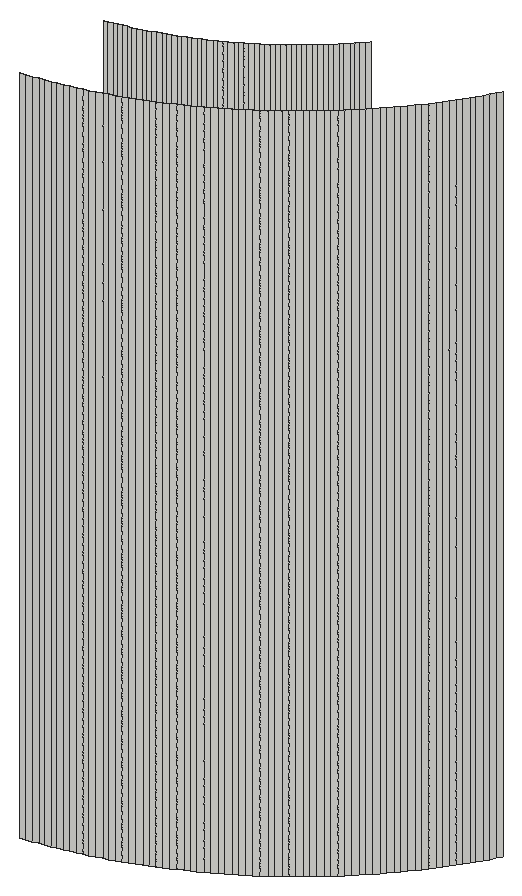
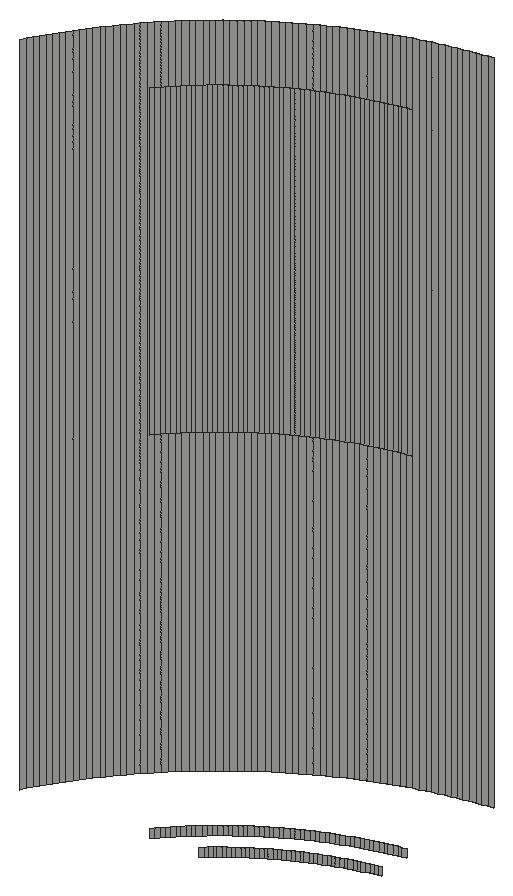
# SketchUp Ruby script. Lengths in inches.
U = 1.inch
M = Sketchup.active_model
def pt(a) = Geom::Point3d.new(a.map { |v| v * U })
def face(e, loops, mat)
  f = e.add_face(loops[0].map { |a| pt(a) })
  loops[1..].each { |l| e.add_face(l.map { |a| pt(a) }).erase! }
  f.material = f.back_material = mat if mat
  f
end
# faces: each face lists its corners as indices into pts; further lists are holes
def faces(e, pts, list, mat = nil) = list.each { |f| face(e, (f[0].is_a?(Array) ? f : [f]).map { |l| l.map { |i| pts[i] } }, mat) }
# xy, xz, yz: faces in a plane at the given z, y or x. An outline is a flat list of corners, or four numbers for a rectangle; further outlines are holes
def ring(l) = l.size == 4 ? [[l[0], l[1]], [l[2], l[1]], [l[2], l[3]], [l[0], l[3]]] : l.each_slice(2).to_a
def flat(e, list, mat, &to3) = list.each { |f| face(e, (f[0].is_a?(Array) ? f : [f]).map { |l| ring(l).map { |u, v| to3.(u, v) } }, mat) }
def xy(e, z, list, mat = nil) = flat(e, list, mat) { |x, y| [x, y, z] }
def xz(e, y, list, mat = nil) = flat(e, list, mat) { |x, z| [x, y, z] }
def yz(e, x, list, mat = nil) = flat(e, list, mat) { |y, z| [x, y, z] }
def lines(e, pts, list) = list.each { |a, b| e.add_line(pt(pts[a]), pt(pts[b])) }
# prism: a flat outline (further loops are holes) pulled along v
def prism(e, loops, v, mat = nil)
  f = face(e, loops, mat); d = Geom::Vector3d.new(v.map { |x| x * U })
  f.pushpull(f.normal.samedirection?(d) ? d.length : -d.length)
end
def box(e, o, s, mat = nil) = prism(e, [[o, [o[0] + s[0], o[1], o[2]], [o[0] + s[0], o[1] + s[1], o[2]], [o[0], o[1] + s[1], o[2]]]], [0, 0, s[2]], mat)
def at(x, y, z, deg = 0) = Geom::Transformation.translation(pt([x, y, z])) * Geom::Transformation.rotation(ORIGIN, Z_AXIS, deg.degrees)
def axes(o, x, y, z) = Geom::Transformation.new([*x, 0, *y, 0, *z, 0, *pt(o).to_a, 1])
def part(name) = M.definitions.add(name)
# library, detail: a bought-in or finely detailed component or shape, given as its bounding box
def library(name, o, s) = part(name).tap { |d| box(d.entities, o, s) }
def detail(e, o, s) = box(e.add_group.entities, o, s)
def put(e, d, t, mat = nil) = e.add_instance(d, t).tap { |i| i.material = mat if mat }
def group(e, t, mat = nil) = e.add_group.tap { |g| g.transformation = t; g.material = mat if mat }.entities
root = M.entities
p = [[327.44,164.25,231],[327.44,164.25,270],[327.13,164.21,270],[327.13,164.21,231],[327.75,164.3,231],[327.75,164.3,270],
  [328.0625,164.35,231],[328.0625,164.35,270],[328.375,164.4,231],[328.375,164.4,270],[328.68,164.46,231],[328.68,164.46,270],
  [328.99,164.52,231],[328.99,164.52,270],[329.3,164.59,231],[329.3,164.59,270],[329.6,164.66,231],[329.6,164.66,270],
  [329.91,164.74,231],[329.91,164.74,270],[330.21,164.82,231],[330.21,164.82,270],[330.51,164.9,231],[330.51,164.9,270],
  [330.82,164.99,231],[330.82,164.99,270],[331.12,165.08,231],[331.12,165.08,270],[331.42,165.17,231],[331.42,165.17,270],
  [331.71,165.27,231],[331.71,165.27,270],[332.01,165.375,231],[332.01,165.375,270],[332.31,165.48,231],[332.31,165.48,270],
  [332.6,165.59,231],[332.6,165.59,270],[332.89,165.71,231],[332.89,165.71,270],[333.18,165.83,231],[333.18,165.83,270],
  [333.47,165.95,231],[333.47,165.95,270],[333.76,166.07,231],[333.76,166.07,270],[334.05,166.2,231],[334.05,166.2,270],
  [334.33,166.34,231],[334.33,166.34,270],[334.61,166.48,231],[334.61,166.48,270],[334.9,166.62,231],[334.9,166.62,270],
  [335.17,166.76,231],[335.17,166.76,270],[335.45,166.91,231],[335.45,166.91,270],[335.73,167.06,231],[335.73,167.06,270],
  [336,167.22,231],[336,167.22,270],[336.27,167.375,231],[336.27,167.375,270],[336.54,167.54,231],[336.54,167.54,270],
  [336.81,167.7,231],[336.81,167.7,270],[337.07,167.87,231],[337.07,167.87,270],[337.33,168.04,231],[337.33,168.04,270],
  [337.59,168.22,231],[337.59,168.22,270],[337.85,168.4,231],[337.85,168.4,270],[338.11,168.58,231],[338.11,168.58,270],
  [338.36,168.77,231],[338.36,168.77,270],[338.61,168.96,231],[338.61,168.96,270],[338.86,169.15,231],[338.86,169.15,270],
  [339.1,169.35,231],[339.1,169.35,270],[339.35,169.55,231],[339.35,169.55,270],[339.59,169.75,231],[339.59,169.75,270],
  [339.82,169.96,231],[339.82,169.96,270],[340.06,170.16,231],[340.06,170.16,270],[340.29,170.375,231],[340.29,170.375,270],
  [327.51,170.35,231],[327.28,170.3,231],[327.28,170.3,231.5],[327.51,170.35,231.5],[327.74,170.39,231],[327.74,170.39,231.5],
  [327.97,170.44,231],[327.97,170.44,231.5],[328.2,170.5,231],[328.2,170.5,231.5],[340.52,170.59,231],[340.52,170.59,270],
  [328.43,170.55,231],[328.43,170.55,231.5],[328.66,170.61,231],[328.66,170.61,231.5],[328.89,170.68,231],[328.89,170.68,231.5],
  [340.75,170.81,231],[340.75,170.81,270],[329.11,170.74,231],[329.11,170.74,231.5],[329.34,170.81,231],[329.34,170.81,231.5],
  [329.5625,170.88,231],[329.5625,170.88,231.5],[340.97,171.03,231],[340.97,171.03,270],[329.79,170.96,231],[329.79,170.96,231.5],
  [330.01,171.03,231],[330.01,171.03,231.5],[330.23,171.11,231],[330.23,171.11,231.5],[341.19,171.25,231],[341.19,171.25,270],
  [330.45,171.2,231],[330.45,171.2,231.5],[330.67,171.28,231],[330.67,171.28,231.5],[330.89,171.37,231],[330.89,171.37,231.5],
  [341.41,171.48,231],[341.41,171.48,270],[331.11,171.46,231],[331.11,171.46,231.5],[331.32,171.56,231],[331.32,171.56,231.5],
  [341.625,171.71,231],[341.625,171.71,270],[331.54,171.65,231],[331.54,171.65,231.5],[331.75,171.75,231],[331.75,171.75,231.5],
  [341.84,171.94,231],[341.84,171.94,270],[331.96,171.86,231],[331.96,171.86,231.5],[332.17,171.96,231],[332.17,171.96,231.5],
  [342.04,172.18,231],[342.04,172.18,270],[332.38,172.07,231],[332.38,172.07,231.5],[332.59,172.18,231],[332.59,172.18,231.5],
  [332.8,172.3,231],[332.8,172.3,231.5],[342.25,172.41,231],[342.25,172.41,270],[327.12,172.31,231],[327.33,172.35,231],
  [327.33,172.35,231.5],[327.12,172.31,231.5],[327.53,172.39,231],[327.53,172.39,231.5],[333,172.41,231],[333,172.41,231.5],
  [327.74,172.44,231],[327.74,172.44,231.5],[327.9375,172.49,231],[327.9375,172.49,231.5],[333.2,172.53,231],[333.2,172.53,231.5],
  [342.45,172.65,231],[342.45,172.65,270],[328.14,172.55,231],[328.14,172.55,231.5],[328.34,172.6,231],[328.34,172.6,231.5],
  [333.4,172.65,231],[333.4,172.65,231.5],[328.54,172.66,231],[328.54,172.66,231.5],[328.74,172.72,231],[328.74,172.72,231.5],
  [328.94,172.78,231],[328.94,172.78,231.5],[333.61,172.78,231],[333.61,172.78,231.5],[342.65,172.9,231],[342.65,172.9,270],
  [329.14,172.85,231],[329.14,172.85,231.5],[329.34,172.92,231],[329.34,172.92,231.5],[333.8,172.9,231],[333.8,172.9,231.5],
  [329.54,172.99,231],[329.54,172.99,231.5],[334,173.03,231],[334,173.03,231.5],[342.85,173.14,231],[342.85,173.14,270],
  [329.73,173.0625,231],[329.73,173.0625,231.5],[334.2,173.17,231],[334.2,173.17,231.5],[329.93,173.14,231],[329.93,173.14,231.5],
  [330.12,173.22,231],[330.12,173.22,231.5],[343.04,173.39,231],[343.04,173.39,270],[330.32,173.3,231],[330.32,173.3,231.5],
  [334.39,173.3,231],[334.39,173.3,231.5],[330.51,173.38,231],[330.51,173.38,231.5],[334.58,173.4375,231],[334.58,173.4375,231.5],
  [330.7,173.47,231],[330.7,173.47,231.5],[334.77,173.58,231],[334.77,173.58,231.5],[343.23,173.64,231],[343.23,173.64,270],
  [330.89,173.56,231],[330.89,173.56,231.5],[331.08,173.65,231],[331.08,173.65,231.5],[334.96,173.72,231],[334.96,173.72,231.5],
  [343.42,173.89,231],[343.42,173.89,270],[331.26,173.74,231],[331.26,173.74,231.5],[331.45,173.84,231],[331.45,173.84,231.5],
  [335.14,173.86,231],[335.14,173.86,231.5],[331.63,173.9375,231],[331.63,173.9375,231.5],[331.82,174.04,231],[331.82,174.04,231.5],
  [335.33,174.01,231],[335.33,174.01,231.5],[343.6,174.15,231],[343.6,174.15,270],[332,174.14,231],[332,174.14,231.5],
  [335.51,174.16,231],[335.51,174.16,231.5],[332.18,174.25,231],[332.18,174.25,231.5],[343.78,174.41,231],[343.78,174.41,270],
  [332.36,174.36,231],[332.36,174.36,231.5],[335.69,174.3125,231],[335.69,174.3125,231.5],[335.87,174.47,231],[335.87,174.47,231.5],
  [332.54,174.47,231],[332.54,174.47,231.5],[343.96,174.67,231],[343.96,174.67,270],[332.71,174.58,231],[332.71,174.58,231.5],
  [336.04,174.625,231],[336.04,174.625,231.5],[332.89,174.7,231],[332.89,174.7,231.5],[336.22,174.78,231],[336.22,174.78,231.5],
  [333.0625,174.8125,231],[333.0625,174.8125,231.5],[344.13,174.93,231],[344.13,174.93,270],[333.23,174.93,231],[333.23,174.93,231.5],
  [336.39,174.94,231],[336.39,174.94,231.5],[333.4,175.06,231],[333.4,175.06,231.5],[336.56,175.11,231],[336.56,175.11,231.5],
  [344.3,175.19,231],[344.3,175.19,270],[333.57,175.18,231],[333.57,175.18,231.5],[336.73,175.27,231],[336.73,175.27,231.5],
  [333.74,175.31,231],[333.74,175.31,231.5],[344.46,175.46,231],[344.46,175.46,270],[333.91,175.43,231],[333.91,175.43,231.5],
  [336.89,175.44,231],[336.89,175.44,231.5],[334.07,175.57,231],[334.07,175.57,231.5],[337.06,175.61,231],[337.06,175.61,231.5],
  [344.625,175.73,231],[344.625,175.73,270],[334.23,175.7,231],[334.23,175.7,231.5],[337.22,175.78,231],[337.22,175.78,231.5],
  [334.39,175.83,231],[334.39,175.83,231.5],[344.78,176,231],[344.78,176,270],[334.55,175.97,231],[334.55,175.97,231.5],
  [337.375,175.96,231],[337.375,175.96,231.5],[334.71,176.11,231],[334.71,176.11,231.5],[337.53,176.13,231],[337.53,176.13,231.5],
  [344.94,176.27,231],[344.94,176.27,270],[327.28,170.3,252],[327.05,170.26,252],[327.05,170.26,270],[327.28,170.3,270],
  [327.51,170.35,252],[327.51,170.35,270],[327.74,170.39,252],[327.74,170.39,270],[327.97,170.44,252],[327.97,170.44,270],
  [328.2,170.5,252],[328.2,170.5,270],[328.43,170.55,252],[328.43,170.55,270],[328.66,170.61,252],[328.66,170.61,270],
  [328.89,170.68,252],[328.89,170.68,270],[329.11,170.74,252],[329.11,170.74,270],[329.34,170.81,252],[329.34,170.81,270],
  [329.5625,170.88,252],[329.5625,170.88,270],[329.79,170.96,252],[329.79,170.96,270],[330.01,171.03,252],[330.01,171.03,270],
  [330.23,171.11,252],[330.23,171.11,270],[330.45,171.2,252],[330.45,171.2,270],[330.67,171.28,252],[330.67,171.28,270],
  [330.89,171.37,252],[330.89,171.37,270],[331.11,171.46,252],[331.11,171.46,270],[331.32,171.56,252],[331.32,171.56,270],
  [331.54,171.65,252],[331.54,171.65,270],[331.75,171.75,252],[331.75,171.75,270],[331.96,171.86,252],[331.96,171.86,270],
  [332.17,171.96,252],[332.17,171.96,270],[332.38,172.07,252],[332.38,172.07,270],[332.59,172.18,252],[332.59,172.18,270],
  [332.8,172.3,252],[332.8,172.3,270],[333,172.41,252],[333,172.41,270],[333.2,172.53,252],[333.2,172.53,270],
  [333.4,172.65,252],[333.4,172.65,270],[333.61,172.78,252],[333.61,172.78,270],[333.8,172.9,252],[333.8,172.9,270],
  [334,173.03,252],[334,173.03,270],[334.2,173.17,252],[334.2,173.17,270],[334.39,173.3,252],[334.39,173.3,270],
  [334.58,173.4375,252],[334.58,173.4375,270],[334.77,173.58,252],[334.77,173.58,270],[334.96,173.72,252],[334.96,173.72,270],
  [335.14,173.86,252],[335.14,173.86,270],[335.33,174.01,252],[335.33,174.01,270],[335.51,174.16,252],[335.51,174.16,270],
  [335.69,174.3125,252],[335.69,174.3125,270],[335.87,174.47,252],[335.87,174.47,270],[336.04,174.625,252],[336.04,174.625,270],
  [336.22,174.78,252],[336.22,174.78,270],[336.39,174.94,252],[336.39,174.94,270],[336.56,175.11,252],[336.56,175.11,270],
  [336.73,175.27,252],[336.73,175.27,270],[336.89,175.44,252],[336.89,175.44,270],[337.06,175.61,252],[337.06,175.61,270],
  [337.22,175.78,252],[337.22,175.78,270],[337.375,175.96,252],[337.375,175.96,270],[337.53,176.13,252],[337.53,176.13,270]]
faces(root,p,[[0,1,2,3],[4,5,1,0],[6,7,5,4],[8,9,7,6],[10,11,9,8],[12,13,11,10],[14,15,13,12],[16,17,15,14],
  [18,19,17,16],[20,21,19,18],[22,23,21,20],[24,25,23,22],[26,27,25,24],[28,29,27,26],[30,31,29,28],[32,33,31,30],
  [34,35,33,32],[36,37,35,34],[38,39,37,36],[40,41,39,38],[42,43,41,40],[44,45,43,42],[46,47,45,44],[48,49,47,46],
  [50,51,49,48],[52,53,51,50],[54,55,53,52],[56,57,55,54],[58,59,57,56],[60,61,59,58],[62,63,61,60],[64,65,63,62],
  [66,67,65,64],[68,69,67,66],[70,71,69,68],[72,73,71,70],[74,75,73,72],[76,77,75,74],[78,79,77,76],[80,81,79,78],
  [82,83,81,80],[84,85,83,82],[86,87,85,84],[88,89,87,86],[90,91,89,88],[92,93,91,90],[94,95,93,92],[96,97,98,99],
  [100,96,99,101],[102,100,101,103],[104,102,103,105],[106,107,95,94],[108,104,105,109],[110,108,109,111],[112,110,111,113],[114,115,107,106],
  [116,112,113,117],[118,116,117,119],[120,118,119,121],[122,123,115,114],[124,120,121,125],[126,124,125,127],[128,126,127,129],[130,131,123,122],
  [132,128,129,133],[134,132,133,135],[136,134,135,137],[138,139,131,130],[140,136,137,141],[142,140,141,143],[144,145,139,138],[146,142,143,147],
  [148,146,147,149],[150,151,145,144],[152,148,149,153],[154,152,153,155],[156,157,151,150],[158,154,155,159],[160,158,159,161],[162,160,161,163],
  [164,165,157,156],[166,167,168,169],[167,170,171,168],[172,162,163,173],[170,174,175,171],[174,176,177,175],[178,172,173,179],[180,181,165,164],
  [176,182,183,177],[182,184,185,183],[186,178,179,187],[184,188,189,185],[188,190,191,189],[190,192,193,191],[194,186,187,195],[196,197,181,180],
  [192,198,199,193],[198,200,201,199],[202,194,195,203],[200,204,205,201],[206,202,203,207],[208,209,197,196],[204,210,211,205],[212,206,207,213],
  [210,214,215,211],[214,216,217,215],[218,219,209,208],[216,220,221,217],[222,212,213,223],[220,224,225,221],[226,222,223,227],[224,228,229,225],
  [230,226,227,231],[232,233,219,218],[228,234,235,229],[234,236,237,235],[238,230,231,239],[240,241,233,232],[236,242,243,237],[242,244,245,243],
  [246,238,239,247],[244,248,249,245],[248,250,251,249],[252,246,247,253],[254,255,241,240],[250,256,257,251],[258,252,253,259],[256,260,261,257],
  [262,263,255,254],[260,264,265,261],[266,258,259,267],[268,266,267,269],[264,270,271,265],[272,273,263,262],[270,274,275,271],[276,268,269,277],
  [274,278,279,275],[280,276,277,281],[278,282,283,279],[284,285,273,272],[282,286,287,283],[288,280,281,289],[286,290,291,287],[292,288,289,293],
  [294,295,285,284],[290,296,297,291],[298,292,293,299],[296,300,301,297],[302,303,295,294],[300,304,305,301],[306,298,299,307],[304,308,309,305],
  [310,306,307,311],[312,313,303,302],[308,314,315,309],[316,310,311,317],[314,318,319,315],[320,321,313,312],[318,322,323,319],[324,316,317,325],
  [322,326,327,323],[328,324,325,329],[330,331,321,320],[332,333,334,335],[336,332,335,337],[338,336,337,339],[340,338,339,341],[342,340,341,343],
  [344,342,343,345],[346,344,345,347],[348,346,347,349],[350,348,349,351],[352,350,351,353],[354,352,353,355],[356,354,355,357],[358,356,357,359],
  [360,358,359,361],[362,360,361,363],[364,362,363,365],[366,364,365,367],[368,366,367,369],[370,368,369,371],[372,370,371,373],[374,372,373,375],
  [376,374,375,377],[378,376,377,379],[380,378,379,381],[382,380,381,383],[384,382,383,385],[386,384,385,387],[388,386,387,389],[390,388,389,391],
  [392,390,391,393],[394,392,393,395],[396,394,395,397],[398,396,397,399],[400,398,399,401],[402,400,401,403],[404,402,403,405],[406,404,405,407],
  [408,406,407,409],[410,408,409,411],[412,410,411,413],[414,412,413,415],[416,414,415,417],[418,416,417,419],[420,418,419,421],[422,420,421,423],
  [424,422,423,425],[426,424,425,427],[428,426,427,429],[430,428,429,431],[432,430,431,433],[434,432,433,435],[436,434,435,437]])
